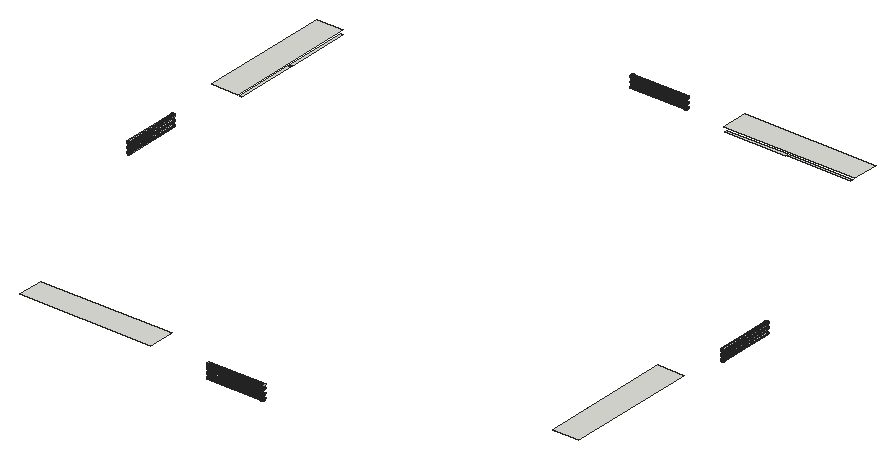
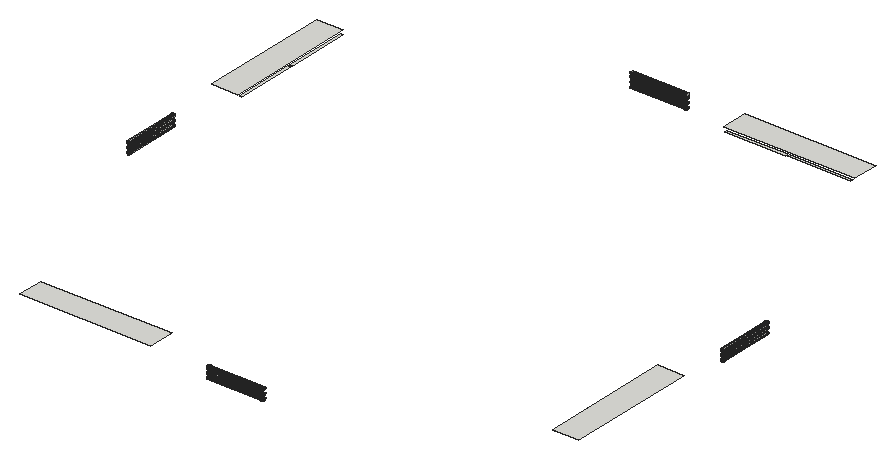
# SketchUp Ruby script. Lengths in inches.
U = 1.inch
M = Sketchup.active_model
def pt(a) = Geom::Point3d.new(a.map { |v| v * U })
def face(e, loops, mat)
  f = e.add_face(loops[0].map { |a| pt(a) })
  loops[1..].each { |l| e.add_face(l.map { |a| pt(a) }).erase! }
  f.material = f.back_material = mat if mat
  f
end
# faces: each face lists its corners as indices into pts; further lists are holes
def faces(e, pts, list, mat = nil) = list.each { |f| face(e, (f[0].is_a?(Array) ? f : [f]).map { |l| l.map { |i| pts[i] } }, mat) }
# xy, xz, yz: faces in a plane at the given z, y or x. An outline is a flat list of corners, or four numbers for a rectangle; further outlines are holes
def ring(l) = l.size == 4 ? [[l[0], l[1]], [l[2], l[1]], [l[2], l[3]], [l[0], l[3]]] : l.each_slice(2).to_a
def flat(e, list, mat, &to3) = list.each { |f| face(e, (f[0].is_a?(Array) ? f : [f]).map { |l| ring(l).map { |u, v| to3.(u, v) } }, mat) }
def xy(e, z, list, mat = nil) = flat(e, list, mat) { |x, y| [x, y, z] }
def xz(e, y, list, mat = nil) = flat(e, list, mat) { |x, z| [x, y, z] }
def yz(e, x, list, mat = nil) = flat(e, list, mat) { |y, z| [x, y, z] }
def lines(e, pts, list) = list.each { |a, b| e.add_line(pt(pts[a]), pt(pts[b])) }
# prism: a flat outline (further loops are holes) pulled along v
def prism(e, loops, v, mat = nil)
  f = face(e, loops, mat); d = Geom::Vector3d.new(v.map { |x| x * U })
  f.pushpull(f.normal.samedirection?(d) ? d.length : -d.length)
end
def box(e, o, s, mat = nil) = prism(e, [[o, [o[0] + s[0], o[1], o[2]], [o[0] + s[0], o[1] + s[1], o[2]], [o[0], o[1] + s[1], o[2]]]], [0, 0, s[2]], mat)
def at(x, y, z, deg = 0) = Geom::Transformation.translation(pt([x, y, z])) * Geom::Transformation.rotation(ORIGIN, Z_AXIS, deg.degrees)
def axes(o, x, y, z) = Geom::Transformation.new([*x, 0, *y, 0, *z, 0, *pt(o).to_a, 1])
def part(name) = M.definitions.add(name)
# library, detail: a bought-in or finely detailed component or shape, given as its bounding box
def library(name, o, s) = part(name).tap { |d| box(d.entities, o, s) }
def detail(e, o, s) = box(e.add_group.entities, o, s)
def put(e, d, t, mat = nil) = e.add_instance(d, t).tap { |i| i.material = mat if mat }
def group(e, t, mat = nil) = e.add_group.tap { |g| g.transformation = t; g.material = mat if mat }.entities
root = M.entities
xy(root,1056.625,[[312.65,102.8125,473.9375,108.8125],[479.9375,102.8125,635.22,108.8125],[1476,277.47,1482,438.75],[1476,444.75,1482,600.03],[138,949.59,144,1104.875],
  [138,1110.875,144,1272.16],[984.78,1440.8125,1140.0625,1446.8125],[1146.0625,1440.8125,1307.35,1446.8125]])
xy(root,1062.625,[[306.65,36.8125,641.22,102.8125],[1482,271.47,1548,606.03],[72,943.59,138,1278.16],[978.78,1446.8125,1313.35,1512.8125]])
yz(root,778.64,[[48.34,1062.02,49.29,1062.14,50.18,1062.51,50.95,1063.1,51.53,1063.86,51.9,1064.75,52.03,1065.7,51.9,1066.66,51.8,1066.89,44.875,1066.89,44.78,1066.66,44.65,1065.7,44.78,1064.75,45.15,1063.86,45.73,1063.1,46.5,1062.51,47.38,1062.14]])
yz(root,922.01,[[48.34,1062.02,47.38,1062.14,46.5,1062.51,45.73,1063.1,45.15,1063.86,44.78,1064.75,44.65,1065.7,44.78,1066.66,44.875,1066.89,51.8,1066.89,51.9,1066.66,52.03,1065.7,51.9,1064.75,51.53,1063.86,50.95,1063.1,50.18,1062.51,49.29,1062.14]])
p = [[922.01,48.34,1029.02],[922.01,47.38,1029.14],[778.64,47.38,1029.14],[778.64,48.34,1029.02],[922.01,49.29,1029.14],[778.64,49.29,1029.14],
  [83.53,662.8,1029.02],[82.57,662.8,1029.14],[82.57,806.17,1029.14],[83.53,806.17,1029.02],[84.48,662.8,1029.14],[84.48,806.17,1029.14],
  [1535.52,886.83,1029.14],[1536.47,886.83,1029.02],[1536.47,743.45,1029.02],[1535.52,743.45,1029.14],[1537.43,886.83,1029.14],[1537.43,743.45,1029.14],
  [697.99,1500.33,1029.14],[697.99,1501.28,1029.02],[841.36,1501.28,1029.02],[841.36,1500.33,1029.14],[697.99,1502.24,1029.14],[841.36,1502.24,1029.14],
  [922.01,46.5,1029.51],[778.64,46.5,1029.51],[922.01,50.18,1029.51],[778.64,50.18,1029.51],[81.68,662.8,1029.51],[81.68,806.17,1029.51],
  [85.37,662.8,1029.51],[85.37,806.17,1029.51],[1534.63,886.83,1029.51],[1534.63,743.45,1029.51],[1538.32,886.83,1029.51],[1538.32,743.45,1029.51],
  [697.99,1499.44,1029.51],[841.36,1499.44,1029.51],[697.99,1503.13,1029.51],[841.36,1503.13,1029.51],[922.01,45.73,1030.1],[778.64,45.73,1030.1],
  [922.01,50.95,1030.1],[778.64,50.95,1030.1],[80.92,662.8,1030.1],[80.92,806.17,1030.1],[86.13,662.8,1030.1],[86.13,806.17,1030.1],
  [1533.87,886.83,1030.1],[1533.87,743.45,1030.1],[1539.08,886.83,1030.1],[1539.08,743.45,1030.1],[697.99,1498.68,1030.1],[841.36,1498.68,1030.1],
  [697.99,1503.89,1030.1],[841.36,1503.89,1030.1],[922.01,45.15,1030.86],[778.64,45.15,1030.86],[922.01,51.53,1030.86],[778.64,51.53,1030.86],
  [80.33,662.8,1030.86],[80.33,806.17,1030.86],[86.72,662.8,1030.86],[86.72,806.17,1030.86],[1533.28,886.83,1030.86],[1533.28,743.45,1030.86],
  [1539.67,886.83,1030.86],[1539.67,743.45,1030.86],[697.99,1498.09,1030.86],[841.36,1498.09,1030.86],[697.99,1504.48,1030.86],[841.36,1504.48,1030.86],
  [922.01,44.78,1031.75],[778.64,44.78,1031.75],[922.01,51.9,1031.75],[778.64,51.9,1031.75],[79.97,662.8,1031.75],[79.97,806.17,1031.75],
  [87.09,662.8,1031.75],[87.09,806.17,1031.75],[1532.91,886.83,1031.75],[1532.91,743.45,1031.75],[1540.03,886.83,1031.75],[1540.03,743.45,1031.75],
  [697.99,1497.72,1031.75],[841.36,1497.72,1031.75],[697.99,1504.85,1031.75],[841.36,1504.85,1031.75],[922.01,44.65,1032.7],[778.64,44.65,1032.7],
  [922.01,52.03,1032.7],[778.64,52.03,1032.7],[79.84,662.8,1032.7],[79.84,806.17,1032.7],[87.21,662.8,1032.7],[87.21,806.17,1032.7],
  [1532.79,886.83,1032.7],[1532.79,743.45,1032.7],[1540.16,886.83,1032.7],[1540.16,743.45,1032.7],[697.99,1497.6,1032.7],[841.36,1497.6,1032.7],
  [697.99,1504.97,1032.7],[841.36,1504.97,1032.7],[922.01,44.78,1033.66],[778.64,44.78,1033.66],[922.01,51.9,1033.66],[778.64,51.9,1033.66],
  [79.97,662.8,1033.66],[79.97,806.17,1033.66],[87.09,662.8,1033.66],[87.09,806.17,1033.66],[1532.91,886.83,1033.66],[1532.91,743.45,1033.66],
  [1540.03,886.83,1033.66],[1540.03,743.45,1033.66],[697.99,1497.72,1033.66],[841.36,1497.72,1033.66],[697.99,1504.85,1033.66],[841.36,1504.85,1033.66],
  [922.01,45.15,1034.55],[778.64,45.15,1034.55],[922.01,51.53,1034.55],[778.64,51.53,1034.55],[80.33,662.8,1034.55],[80.33,806.17,1034.55],
  [86.72,662.8,1034.55],[86.72,806.17,1034.55],[1533.28,886.83,1034.55],[1533.28,743.45,1034.55],[1539.67,886.83,1034.55],[1539.67,743.45,1034.55],
  [697.99,1498.09,1034.55],[841.36,1498.09,1034.55],[697.99,1504.48,1034.55],[841.36,1504.48,1034.55],[922.01,45.73,1035.3125],[778.64,45.73,1035.3125],
  [922.01,50.95,1035.3125],[778.64,50.95,1035.3125],[80.92,662.8,1035.3125],[80.92,806.17,1035.3125],[86.13,662.8,1035.3125],[86.13,806.17,1035.3125],
  [1533.87,886.83,1035.3125],[1533.87,743.45,1035.3125],[1539.08,886.83,1035.3125],[1539.08,743.45,1035.3125],[697.99,1498.68,1035.3125],[841.36,1498.68,1035.3125],
  [697.99,1503.89,1035.3125],[841.36,1503.89,1035.3125],[922.01,46.5,1035.9],[778.64,46.5,1035.9],[922.01,50.18,1035.9],[778.64,50.18,1035.9],
  [81.68,662.8,1035.9],[81.68,806.17,1035.9],[85.37,662.8,1035.9],[85.37,806.17,1035.9],[1534.63,886.83,1035.9],[1534.63,743.45,1035.9],
  [1538.32,886.83,1035.9],[1538.32,743.45,1035.9],[697.99,1499.44,1035.9],[841.36,1499.44,1035.9],[697.99,1503.13,1035.9],[841.36,1503.13,1035.9],
  [922.01,47.38,1036.27],[778.64,47.38,1036.27],[922.01,49.29,1036.27],[778.64,49.29,1036.27],[82.57,662.8,1036.27],[82.57,806.17,1036.27],
  [84.48,662.8,1036.27],[84.48,806.17,1036.27],[1535.52,886.83,1036.27],[1535.52,743.45,1036.27],[1537.43,886.83,1036.27],[1537.43,743.45,1036.27],
  [697.99,1500.33,1036.27],[841.36,1500.33,1036.27],[697.99,1502.24,1036.27],[841.36,1502.24,1036.27],[922.01,48.34,1036.39],[778.64,48.34,1036.39],
  [83.53,662.8,1036.39],[83.53,806.17,1036.39],[1536.47,886.83,1036.39],[1536.47,743.45,1036.39],[697.99,1501.28,1036.39],[841.36,1501.28,1036.39],
  [922.01,48.34,1041.02],[922.01,47.38,1041.14],[778.64,47.38,1041.14],[778.64,48.34,1041.02],[922.01,49.29,1041.14],[778.64,49.29,1041.14],
  [83.53,662.8,1041.02],[82.57,662.8,1041.14],[82.57,806.17,1041.14],[83.53,806.17,1041.02],[84.48,662.8,1041.14],[84.48,806.17,1041.14],
  [1535.52,886.83,1041.14],[1536.47,886.83,1041.02],[1536.47,743.45,1041.02],[1535.52,743.45,1041.14],[1537.43,886.83,1041.14],[1537.43,743.45,1041.14],
  [697.99,1500.33,1041.14],[697.99,1501.28,1041.02],[841.36,1501.28,1041.02],[841.36,1500.33,1041.14],[697.99,1502.24,1041.14],[841.36,1502.24,1041.14],
  [922.01,46.5,1041.51],[778.64,46.5,1041.51],[922.01,50.18,1041.51],[778.64,50.18,1041.51],[81.68,662.8,1041.51],[81.68,806.17,1041.51],
  [85.37,662.8,1041.51],[85.37,806.17,1041.51],[1534.63,886.83,1041.51],[1534.63,743.45,1041.51],[1538.32,886.83,1041.51],[1538.32,743.45,1041.51],
  [697.99,1499.44,1041.51],[841.36,1499.44,1041.51],[697.99,1503.13,1041.51],[841.36,1503.13,1041.51],[922.01,45.73,1042.1],[778.64,45.73,1042.1],
  [922.01,50.95,1042.1],[778.64,50.95,1042.1],[80.92,662.8,1042.1],[80.92,806.17,1042.1],[86.13,662.8,1042.1],[86.13,806.17,1042.1],
  [1533.87,886.83,1042.1],[1533.87,743.45,1042.1],[1539.08,886.83,1042.1],[1539.08,743.45,1042.1],[697.99,1498.68,1042.1],[841.36,1498.68,1042.1],
  [697.99,1503.89,1042.1],[841.36,1503.89,1042.1],[922.01,45.15,1042.86],[778.64,45.15,1042.86],[922.01,51.53,1042.86],[778.64,51.53,1042.86],
  [80.33,662.8,1042.86],[80.33,806.17,1042.86],[86.72,662.8,1042.86],[86.72,806.17,1042.86],[1533.28,886.83,1042.86],[1533.28,743.45,1042.86],
  [1539.67,886.83,1042.86],[1539.67,743.45,1042.86],[697.99,1498.09,1042.86],[841.36,1498.09,1042.86],[697.99,1504.48,1042.86],[841.36,1504.48,1042.86],
  [922.01,44.78,1043.75],[778.64,44.78,1043.75],[922.01,51.9,1043.75],[778.64,51.9,1043.75],[79.97,662.8,1043.75],[79.97,806.17,1043.75],
  [87.09,662.8,1043.75],[87.09,806.17,1043.75],[1532.91,886.83,1043.75],[1532.91,743.45,1043.75],[1540.03,886.83,1043.75],[1540.03,743.45,1043.75],
  [697.99,1497.72,1043.75],[841.36,1497.72,1043.75],[697.99,1504.85,1043.75],[841.36,1504.85,1043.75],[922.01,44.65,1044.7],[778.64,44.65,1044.7],
  [922.01,52.03,1044.7],[778.64,52.03,1044.7],[79.84,662.8,1044.7],[79.84,806.17,1044.7],[87.21,662.8,1044.7],[87.21,806.17,1044.7],
  [1532.79,886.83,1044.7],[1532.79,743.45,1044.7],[1540.16,886.83,1044.7],[1540.16,743.45,1044.7],[697.99,1497.6,1044.7],[841.36,1497.6,1044.7],
  [697.99,1504.97,1044.7],[841.36,1504.97,1044.7],[922.01,44.78,1045.66],[778.64,44.78,1045.66],[922.01,51.9,1045.66],[778.64,51.9,1045.66],
  [79.97,662.8,1045.66],[79.97,806.17,1045.66],[87.09,662.8,1045.66],[87.09,806.17,1045.66],[1532.91,886.83,1045.66],[1532.91,743.45,1045.66],
  [1540.03,886.83,1045.66],[1540.03,743.45,1045.66],[697.99,1497.72,1045.66],[841.36,1497.72,1045.66],[697.99,1504.85,1045.66],[841.36,1504.85,1045.66],
  [922.01,45.15,1046.55],[778.64,45.15,1046.55],[922.01,51.53,1046.55],[778.64,51.53,1046.55],[80.33,662.8,1046.55],[80.33,806.17,1046.55],
  [86.72,662.8,1046.55],[86.72,806.17,1046.55],[1533.28,886.83,1046.55],[1533.28,743.45,1046.55],[1539.67,886.83,1046.55],[1539.67,743.45,1046.55],
  [697.99,1498.09,1046.55],[841.36,1498.09,1046.55],[697.99,1504.48,1046.55],[841.36,1504.48,1046.55],[922.01,45.73,1047.3125],[778.64,45.73,1047.3125],
  [922.01,50.95,1047.3125],[778.64,50.95,1047.3125],[80.92,662.8,1047.3125],[80.92,806.17,1047.3125],[86.13,662.8,1047.3125],[86.13,806.17,1047.3125],
  [1533.87,886.83,1047.3125],[1533.87,743.45,1047.3125],[1539.08,886.83,1047.3125],[1539.08,743.45,1047.3125],[697.99,1498.68,1047.3125],[841.36,1498.68,1047.3125],
  [697.99,1503.89,1047.3125],[841.36,1503.89,1047.3125],[922.01,46.5,1047.9],[778.64,46.5,1047.9],[922.01,50.18,1047.9],[778.64,50.18,1047.9],
  [81.68,662.8,1047.9],[81.68,806.17,1047.9],[85.37,662.8,1047.9],[85.37,806.17,1047.9],[1534.63,886.83,1047.9],[1534.63,743.45,1047.9],
  [1538.32,886.83,1047.9],[1538.32,743.45,1047.9],[697.99,1499.44,1047.9],[841.36,1499.44,1047.9],[697.99,1503.13,1047.9],[841.36,1503.13,1047.9],
  [922.01,47.38,1048.27],[778.64,47.38,1048.27],[922.01,49.29,1048.27],[778.64,49.29,1048.27],[82.57,662.8,1048.27],[82.57,806.17,1048.27],
  [84.48,662.8,1048.27],[84.48,806.17,1048.27],[1535.52,886.83,1048.27],[1535.52,743.45,1048.27],[1537.43,886.83,1048.27],[1537.43,743.45,1048.27],
  [697.99,1500.33,1048.27],[841.36,1500.33,1048.27],[697.99,1502.24,1048.27],[841.36,1502.24,1048.27],[922.01,48.34,1048.39],[778.64,48.34,1048.39],
  [83.53,662.8,1048.39],[83.53,806.17,1048.39],[1536.47,886.83,1048.39],[1536.47,743.45,1048.39],[697.99,1501.28,1048.39],[841.36,1501.28,1048.39],
  [922.01,48.34,1053.02],[922.01,47.38,1053.14],[778.64,47.38,1053.14],[778.64,48.34,1053.02],[922.01,49.29,1053.14],[778.64,49.29,1053.14],
  [83.53,662.8,1053.02],[82.57,662.8,1053.14],[82.57,806.17,1053.14],[83.53,806.17,1053.02],[84.48,662.8,1053.14],[84.48,806.17,1053.14],
  [1535.52,886.83,1053.14],[1536.47,886.83,1053.02],[1536.47,743.45,1053.02],[1535.52,743.45,1053.14],[1537.43,886.83,1053.14],[1537.43,743.45,1053.14],
  [697.99,1500.33,1053.14],[697.99,1501.28,1053.02],[841.36,1501.28,1053.02],[841.36,1500.33,1053.14],[697.99,1502.24,1053.14],[841.36,1502.24,1053.14],
  [922.01,46.5,1053.51],[778.64,46.5,1053.51],[922.01,50.18,1053.51],[778.64,50.18,1053.51],[81.68,662.8,1053.51],[81.68,806.17,1053.51],
  [85.37,662.8,1053.51],[85.37,806.17,1053.51],[1534.63,886.83,1053.51],[1534.63,743.45,1053.51],[1538.32,886.83,1053.51],[1538.32,743.45,1053.51],
  [697.99,1499.44,1053.51],[841.36,1499.44,1053.51],[697.99,1503.13,1053.51],[841.36,1503.13,1053.51],[922.01,45.73,1054.1],[778.64,45.73,1054.1],
  [922.01,50.95,1054.1],[778.64,50.95,1054.1],[80.92,662.8,1054.1],[80.92,806.17,1054.1],[86.13,662.8,1054.1],[86.13,806.17,1054.1],
  [1533.87,886.83,1054.1],[1533.87,743.45,1054.1],[1539.08,886.83,1054.1],[1539.08,743.45,1054.1],[697.99,1498.68,1054.1],[841.36,1498.68,1054.1],
  [697.99,1503.89,1054.1],[841.36,1503.89,1054.1],[922.01,45.15,1054.86],[778.64,45.15,1054.86],[922.01,51.53,1054.86],[778.64,51.53,1054.86],
  [80.33,662.8,1054.86],[80.33,806.17,1054.86],[86.72,662.8,1054.86],[86.72,806.17,1054.86],[1533.28,886.83,1054.86],[1533.28,743.45,1054.86],
  [1539.67,886.83,1054.86],[1539.67,743.45,1054.86],[697.99,1498.09,1054.86],[841.36,1498.09,1054.86],[697.99,1504.48,1054.86],[841.36,1504.48,1054.86],
  [922.01,44.78,1055.75],[778.64,44.78,1055.75],[922.01,51.9,1055.75],[778.64,51.9,1055.75],[79.97,662.8,1055.75],[79.97,806.17,1055.75],
  [87.09,662.8,1055.75],[87.09,806.17,1055.75],[1532.91,886.83,1055.75],[1532.91,743.45,1055.75],[1540.03,886.83,1055.75],[1540.03,743.45,1055.75],
  [697.99,1497.72,1055.75],[841.36,1497.72,1055.75],[697.99,1504.85,1055.75],[841.36,1504.85,1055.75],[922.01,44.65,1056.7],[778.64,44.65,1056.7],
  [922.01,52.03,1056.7],[778.64,52.03,1056.7],[79.84,662.8,1056.7],[79.84,806.17,1056.7],[87.21,662.8,1056.7],[87.21,806.17,1056.7],
  [1532.79,886.83,1056.7],[1532.79,743.45,1056.7],[1540.16,886.83,1056.7],[1540.16,743.45,1056.7],[697.99,1497.6,1056.7],[841.36,1497.6,1056.7],
  [697.99,1504.97,1056.7],[841.36,1504.97,1056.7],[922.01,44.78,1057.66],[778.64,44.78,1057.66],[922.01,51.9,1057.66],[778.64,51.9,1057.66],
  [79.97,662.8,1057.66],[79.97,806.17,1057.66],[87.09,662.8,1057.66],[87.09,806.17,1057.66],[1532.91,886.83,1057.66],[1532.91,743.45,1057.66],
  [1540.03,886.83,1057.66],[1540.03,743.45,1057.66],[697.99,1497.72,1057.66],[841.36,1497.72,1057.66],[697.99,1504.85,1057.66],[841.36,1504.85,1057.66],
  [922.01,45.15,1058.55],[778.64,45.15,1058.55],[922.01,51.53,1058.55],[778.64,51.53,1058.55],[80.33,662.8,1058.55],[80.33,806.17,1058.55],
  [86.72,662.8,1058.55],[86.72,806.17,1058.55],[1533.28,886.83,1058.55],[1533.28,743.45,1058.55],[1539.67,886.83,1058.55],[1539.67,743.45,1058.55],
  [697.99,1498.09,1058.55],[841.36,1498.09,1058.55],[697.99,1504.48,1058.55],[841.36,1504.48,1058.55],[922.01,45.73,1059.3125],[778.64,45.73,1059.3125],
  [922.01,50.95,1059.3125],[778.64,50.95,1059.3125],[80.92,662.8,1059.3125],[80.92,806.17,1059.3125],[86.13,662.8,1059.3125],[86.13,806.17,1059.3125],
  [1533.87,886.83,1059.3125],[1533.87,743.45,1059.3125],[1539.08,886.83,1059.3125],[1539.08,743.45,1059.3125],[697.99,1498.68,1059.3125],[841.36,1498.68,1059.3125],
  [697.99,1503.89,1059.3125],[841.36,1503.89,1059.3125],[922.01,46.5,1059.9],[778.64,46.5,1059.9],[922.01,50.18,1059.9],[778.64,50.18,1059.9],
  [81.68,662.8,1059.9],[81.68,806.17,1059.9],[85.37,662.8,1059.9],[85.37,806.17,1059.9],[1534.63,886.83,1059.9],[1534.63,743.45,1059.9],
  [1538.32,886.83,1059.9],[1538.32,743.45,1059.9],[697.99,1499.44,1059.9],[841.36,1499.44,1059.9],[697.99,1503.13,1059.9],[841.36,1503.13,1059.9],
  [922.01,47.38,1060.27],[778.64,47.38,1060.27],[922.01,49.29,1060.27],[778.64,49.29,1060.27],[82.57,662.8,1060.27],[82.57,806.17,1060.27],
  [84.48,662.8,1060.27],[84.48,806.17,1060.27],[1535.52,886.83,1060.27],[1535.52,743.45,1060.27],[1537.43,886.83,1060.27],[1537.43,743.45,1060.27],
  [697.99,1500.33,1060.27],[841.36,1500.33,1060.27],[697.99,1502.24,1060.27],[841.36,1502.24,1060.27],[922.01,48.34,1060.39],[778.64,48.34,1060.39],
  [83.53,662.8,1060.39],[83.53,806.17,1060.39],[1536.47,886.83,1060.39],[1536.47,743.45,1060.39],[697.99,1501.28,1060.39],[841.36,1501.28,1060.39],
  [922.01,48.34,1062.02],[922.01,47.38,1062.14],[778.64,47.38,1062.14],[778.64,48.34,1062.02],[922.01,49.29,1062.14],[778.64,49.29,1062.14],
  [922.01,46.5,1062.51],[778.64,46.5,1062.51],[922.01,50.18,1062.51],[778.64,50.18,1062.51],[922.01,45.73,1063.1],[778.64,45.73,1063.1],
  [922.01,50.95,1063.1],[778.64,50.95,1063.1],[922.01,45.15,1063.86],[778.64,45.15,1063.86],[922.01,51.53,1063.86],[778.64,51.53,1063.86],
  [922.01,44.78,1064.75],[778.64,44.78,1064.75],[922.01,51.9,1064.75],[778.64,51.9,1064.75],[922.01,44.65,1065.7],[778.64,44.65,1065.7],
  [922.01,52.03,1065.7],[778.64,52.03,1065.7]]
faces(root,p,[[0,1,2,3],[4,0,3,5],[6,7,8,9],[10,6,9,11],[12,13,14,15],[13,16,17,14],[18,19,20,21],[19,22,23,20],
  [1,24,25,2],[26,4,5,27],[7,28,29,8],[30,10,11,31],[32,12,15,33],[16,34,35,17],[36,18,21,37],[22,38,39,23],
  [24,40,41,25],[42,26,27,43],[28,44,45,29],[46,30,31,47],[48,32,33,49],[34,50,51,35],[52,36,37,53],[38,54,55,39],
  [40,56,57,41],[58,42,43,59],[44,60,61,45],[62,46,47,63],[64,48,49,65],[50,66,67,51],[68,52,53,69],[54,70,71,55],
  [56,72,73,57],[74,58,59,75],[60,76,77,61],[78,62,63,79],[80,64,65,81],[66,82,83,67],[84,68,69,85],[70,86,87,71],
  [72,88,89,73],[90,74,75,91],[76,92,93,77],[94,78,79,95],[96,80,81,97],[82,98,99,83],[100,84,85,101],[86,102,103,87],
  [88,104,105,89],[106,90,91,107],[92,108,109,93],[110,94,95,111],[112,96,97,113],[98,114,115,99],[116,100,101,117],[102,118,119,103],
  [104,120,121,105],[122,106,107,123],[108,124,125,109],[126,110,111,127],[128,112,113,129],[114,130,131,115],[132,116,117,133],[118,134,135,119],
  [120,136,137,121],[138,122,123,139],[124,140,141,125],[142,126,127,143],[144,128,129,145],[130,146,147,131],[148,132,133,149],[134,150,151,135],
  [136,152,153,137],[154,138,139,155],[140,156,157,141],[158,142,143,159],[160,144,145,161],[146,162,163,147],[164,148,149,165],[150,166,167,151],
  [152,168,169,153],[170,154,155,171],[156,172,173,157],[174,158,159,175],[176,160,161,177],[162,178,179,163],[180,164,165,181],[166,182,183,167],
  [168,184,185,169],[184,170,171,185],[172,186,187,173],[186,174,175,187],[188,176,177,189],[178,188,189,179],[190,180,181,191],[182,190,191,183],
  [192,193,194,195],[196,192,195,197],[198,199,200,201],[202,198,201,203],[204,205,206,207],[205,208,209,206],[210,211,212,213],[211,214,215,212],
  [193,216,217,194],[218,196,197,219],[199,220,221,200],[222,202,203,223],[224,204,207,225],[208,226,227,209],[228,210,213,229],[214,230,231,215],
  [216,232,233,217],[234,218,219,235],[220,236,237,221],[238,222,223,239],[240,224,225,241],[226,242,243,227],[244,228,229,245],[230,246,247,231],
  [232,248,249,233],[250,234,235,251],[236,252,253,237],[254,238,239,255],[256,240,241,257],[242,258,259,243],[260,244,245,261],[246,262,263,247],
  [248,264,265,249],[266,250,251,267],[252,268,269,253],[270,254,255,271],[272,256,257,273],[258,274,275,259],[276,260,261,277],[262,278,279,263],
  [264,280,281,265],[282,266,267,283],[268,284,285,269],[286,270,271,287],[288,272,273,289],[274,290,291,275],[292,276,277,293],[278,294,295,279],
  [280,296,297,281],[298,282,283,299],[284,300,301,285],[302,286,287,303],[304,288,289,305],[290,306,307,291],[308,292,293,309],[294,310,311,295],
  [296,312,313,297],[314,298,299,315],[300,316,317,301],[318,302,303,319],[320,304,305,321],[306,322,323,307],[324,308,309,325],[310,326,327,311],
  [312,328,329,313],[330,314,315,331],[316,332,333,317],[334,318,319,335],[336,320,321,337],[322,338,339,323],[340,324,325,341],[326,342,343,327],
  [328,344,345,329],[346,330,331,347],[332,348,349,333],[350,334,335,351],[352,336,337,353],[338,354,355,339],[356,340,341,357],[342,358,359,343],
  [344,360,361,345],[362,346,347,363],[348,364,365,349],[366,350,351,367],[368,352,353,369],[354,370,371,355],[372,356,357,373],[358,374,375,359],
  [360,376,377,361],[376,362,363,377],[364,378,379,365],[378,366,367,379],[380,368,369,381],[370,380,381,371],[382,372,373,383],[374,382,383,375],
  [384,385,386,387],[388,384,387,389],[390,391,392,393],[394,390,393,395],[396,397,398,399],[397,400,401,398],[402,403,404,405],[403,406,407,404],
  [385,408,409,386],[410,388,389,411],[391,412,413,392],[414,394,395,415],[416,396,399,417],[400,418,419,401],[420,402,405,421],[406,422,423,407],
  [408,424,425,409],[426,410,411,427],[412,428,429,413],[430,414,415,431],[432,416,417,433],[418,434,435,419],[436,420,421,437],[422,438,439,423],
  [424,440,441,425],[442,426,427,443],[428,444,445,429],[446,430,431,447],[448,432,433,449],[434,450,451,435],[452,436,437,453],[438,454,455,439],
  [440,456,457,441],[458,442,443,459],[444,460,461,445],[462,446,447,463],[464,448,449,465],[450,466,467,451],[468,452,453,469],[454,470,471,455],
  [456,472,473,457],[474,458,459,475],[460,476,477,461],[478,462,463,479],[480,464,465,481],[466,482,483,467],[484,468,469,485],[470,486,487,471],
  [472,488,489,473],[490,474,475,491],[476,492,493,477],[494,478,479,495],[496,480,481,497],[482,498,499,483],[500,484,485,501],[486,502,503,487],
  [488,504,505,489],[506,490,491,507],[492,508,509,493],[510,494,495,511],[512,496,497,513],[498,514,515,499],[516,500,501,517],[502,518,519,503],
  [504,520,521,505],[522,506,507,523],[508,524,525,509],[526,510,511,527],[528,512,513,529],[514,530,531,515],[532,516,517,533],[518,534,535,519],
  [520,536,537,521],[538,522,523,539],[524,540,541,525],[542,526,527,543],[544,528,529,545],[530,546,547,531],[548,532,533,549],[534,550,551,535],
  [536,552,553,537],[554,538,539,555],[540,556,557,541],[558,542,543,559],[560,544,545,561],[546,562,563,547],[564,548,549,565],[550,566,567,551],
  [552,568,569,553],[568,554,555,569],[556,570,571,557],[570,558,559,571],[572,560,561,573],[562,572,573,563],[574,564,565,575],[566,574,575,567],
  [576,577,578,579],[580,576,579,581],[577,582,583,578],[584,580,581,585],[582,586,587,583],[588,584,585,589],[586,590,591,587],[592,588,589,593],
  [590,594,595,591],[596,592,593,597],[594,598,599,595],[600,596,597,601]])
